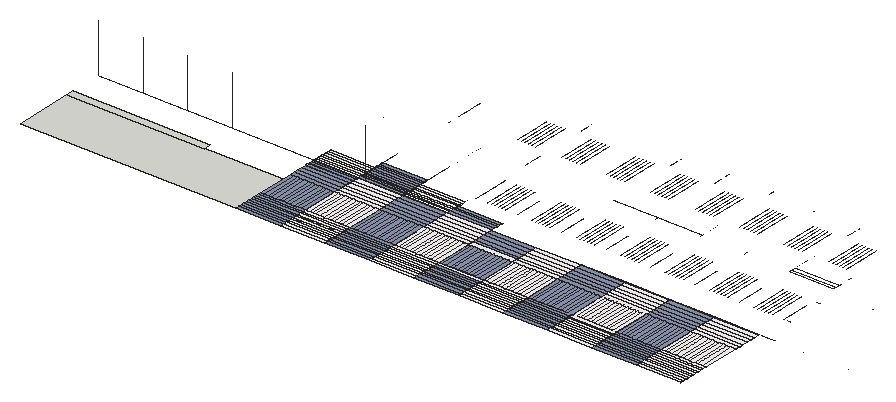
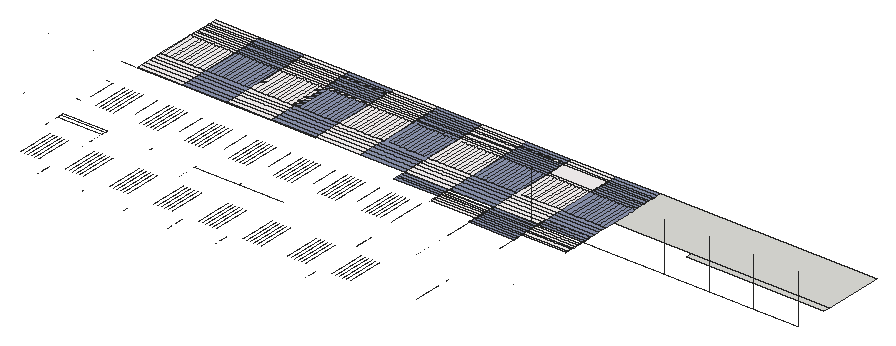
# SketchUp Ruby script. Lengths in inches.
U = 1.inch
M = Sketchup.active_model
def pt(a) = Geom::Point3d.new(a.map { |v| v * U })
def face(e, loops, mat)
  f = e.add_face(loops[0].map { |a| pt(a) })
  loops[1..].each { |l| e.add_face(l.map { |a| pt(a) }).erase! }
  f.material = f.back_material = mat if mat
  f
end
# faces: each face lists its corners as indices into pts; further lists are holes
def faces(e, pts, list, mat = nil) = list.each { |f| face(e, (f[0].is_a?(Array) ? f : [f]).map { |l| l.map { |i| pts[i] } }, mat) }
# xy, xz, yz: faces in a plane at the given z, y or x. An outline is a flat list of corners, or four numbers for a rectangle; further outlines are holes
def ring(l) = l.size == 4 ? [[l[0], l[1]], [l[2], l[1]], [l[2], l[3]], [l[0], l[3]]] : l.each_slice(2).to_a
def flat(e, list, mat, &to3) = list.each { |f| face(e, (f[0].is_a?(Array) ? f : [f]).map { |l| ring(l).map { |u, v| to3.(u, v) } }, mat) }
def xy(e, z, list, mat = nil) = flat(e, list, mat) { |x, y| [x, y, z] }
def xz(e, y, list, mat = nil) = flat(e, list, mat) { |x, z| [x, y, z] }
def yz(e, x, list, mat = nil) = flat(e, list, mat) { |y, z| [x, y, z] }
def lines(e, pts, list) = list.each { |a, b| e.add_line(pt(pts[a]), pt(pts[b])) }
# prism: a flat outline (further loops are holes) pulled along v
def prism(e, loops, v, mat = nil)
  f = face(e, loops, mat); d = Geom::Vector3d.new(v.map { |x| x * U })
  f.pushpull(f.normal.samedirection?(d) ? d.length : -d.length)
end
def box(e, o, s, mat = nil) = prism(e, [[o, [o[0] + s[0], o[1], o[2]], [o[0] + s[0], o[1] + s[1], o[2]], [o[0], o[1] + s[1], o[2]]]], [0, 0, s[2]], mat)
def at(x, y, z, deg = 0) = Geom::Transformation.translation(pt([x, y, z])) * Geom::Transformation.rotation(ORIGIN, Z_AXIS, deg.degrees)
def axes(o, x, y, z) = Geom::Transformation.new([*x, 0, *y, 0, *z, 0, *pt(o).to_a, 1])
def part(name) = M.definitions.add(name)
# library, detail: a bought-in or finely detailed component or shape, given as its bounding box
def library(name, o, s) = part(name).tap { |d| box(d.entities, o, s) }
def detail(e, o, s) = box(e.add_group.entities, o, s)
def put(e, d, t, mat = nil) = e.add_instance(d, t).tap { |i| i.material = mat if mat }
def group(e, t, mat = nil) = e.add_group.tap { |g| g.transformation = t; g.material = mat if mat }.entities
root = M.entities
M.materials.add("Niraj_Shirt").color = [144, 153, 181]
M.materials.add("[0010_Snow]").color = [255, 250, 250]
xy(root,3034.69,[[80.5,1936.0625,635.4,2086.95],[80.5,2086.95,433.875,2104.7]])
xy(root,3034.69,[[635.4,1936.0625,749.59,1945.25],[864.34,1936.0625,978.21,1945.25],[1092.96,1936.0625,1206.84,1945.25],[1321.59,1936.0625,1435.46,1945.25],[1550.21,1936.0625,1664.09,1945.25],
  [635.4,1945.25,749.59,1954.43],[864.34,1945.25,978.21,1954.43],[1092.96,1945.25,1206.84,1954.43],[1321.59,1945.25,1435.46,1954.43],[1550.21,1945.25,1664.09,1954.43],
  [635.4,1954.43,749.59,1961.9375],[864.34,1954.43,978.21,1961.9375],[[1092.84,1954.43,1092.84,1961.9375,1206.84,1961.9375,1206.84,2007.9,1092.84,2007.9,1092.84,2015.89,1092.96,2015.89,1092.96,2124.125,1206.96,2124.125,1206.96,2111.27,1207.15,2111.27,1207.15,1954.43],[1101.05,2015.89,1196.24,2111.27]],[1092.96,1954.43,1206.84,1961.9375],[1321.46,1954.43,1321.46,1961.9375,1435.46,1961.9375,1435.46,2007.9,1321.46,2007.9,1321.46,2015.89,1424.86,2015.89,1424.86,2111.27,1435.59,2111.27,1435.59,2015.89,1435.78,2015.89,1435.78,1954.43],
  [1550.21,1954.43,1664.09,1961.9375],[635.4,1961.9375,749.59,1969.45],[864.34,1961.9375,978.21,1969.45],[1092.96,1961.9375,1206.84,1969.45],[1321.59,1961.9375,1435.46,1969.45],
  [1550.21,1961.9375,1664.09,1969.45],[635.4,1969.45,749.59,1977.23],[864.34,1969.45,978.21,1977.23],[1092.96,1969.45,1206.84,1977.23],[1321.59,1969.45,1435.46,1977.23],
  [1550.21,1969.45,1664.09,1977.23],[635.4,1977.23,749.59,1985.01],[864.34,1977.23,978.21,1985.01],[1092.96,1977.23,1206.84,1985.01],[1321.59,1977.23,1435.46,1985.01],
  [1550.21,1977.23,1664.09,1985.01],[635.4,1985.01,749.59,1992.46],[864.34,1985.01,978.21,1992.46],[1092.96,1985.01,1206.84,1992.46],[1321.59,1985.01,1435.46,1992.46],
  [1550.21,1985.01,1664.09,1992.46],[635.4,1992.46,749.59,1999.91],[864.34,1992.46,978.21,1999.91],[1092.96,1992.46,1206.84,1999.91],[1321.59,1992.46,1435.46,1999.91],
  [1550.21,1992.46,1664.09,1999.91],[635.4,1999.91,749.59,2007.9],[864.34,1999.91,978.21,2007.9],[1092.96,1999.91,1206.84,2007.9],[1321.59,1999.91,1435.46,2007.9],
  [1550.21,1999.91,1664.09,2007.9],[635.4,2007.9,749.59,2015.89],[864.34,2007.9,978.21,2015.89],[1550.21,2007.9,1664.09,2015.89],[635.4,2015.89,643.8,2111.27],
  [643.8,2015.89,652.45,2111.27],[652.45,2015.89,662.47,2111.27],[662.47,2015.89,672.48,2111.27],[672.48,2015.89,682.48,2111.27],[682.48,2015.89,691.13,2111.27],
  [691.13,2015.89,700.68,2111.27],[700.68,2015.89,709.32,2111.27],[709.32,2015.89,719.31,2111.27],[719.31,2015.89,727.95,2111.27],[727.95,2015.89,738.99,2111.27],
  [738.99,2015.89,749.71,2111.27],[864.34,2015.89,872.43,2111.27],[872.43,2015.89,881.08,2111.27],[881.08,2015.89,891.1,2111.27],[891.1,2015.89,901.1,2111.27],
  [901.1,2015.89,911.11,2111.27],[911.11,2015.89,919.76,2111.27],[919.76,2015.89,929.31,2111.27],[929.31,2015.89,937.94,2111.27],[937.94,2015.89,947.93,2111.27],
  [947.93,2015.89,956.58,2111.27],[956.58,2015.89,967.61,2111.27],[967.61,2015.89,978.34,2111.27],[1092.96,2015.89,1101.05,2111.27],[1101.05,2015.89,1109.7,2111.27],
  [1109.7,2015.89,1119.72,2111.27],[1119.72,2015.89,1129.73,2111.27],[1129.73,2015.89,1139.73,2111.27],[1139.73,2015.89,1148.38,2111.27],[1148.38,2015.89,1157.93,2111.27],
  [1157.93,2015.89,1166.57,2111.27],[1166.57,2015.89,1176.56,2111.27],[1176.56,2015.89,1185.2,2111.27],[1185.2,2015.89,1196.24,2111.27],[1196.24,2015.89,1206.96,2111.27],
  [1321.59,2015.89,1329.68,2111.27],[1329.68,2015.89,1338.33,2111.27],[1338.33,2015.89,1348.35,2111.27],[1348.35,2015.89,1358.35,2111.27],[1358.35,2015.89,1368.36,2111.27],
  [1368.36,2015.89,1377.01,2111.27],[1377.01,2015.89,1386.56,2111.27],[1386.56,2015.89,1395.19,2111.27],[1395.19,2015.89,1405.18,2111.27],[1405.18,2015.89,1413.83,2111.27],
  [1413.83,2015.89,1424.86,2111.27],[1550.21,2015.89,1558.3,2111.27],[1558.3,2015.89,1566.95,2111.27],[1566.95,2015.89,1576.97,2111.27],[1576.97,2015.89,1586.98,2111.27],
  [1586.98,2015.89,1596.98,2111.27],[1596.98,2015.89,1605.63,2111.27],[1605.63,2015.89,1615.18,2111.27],[1615.18,2015.89,1623.82,2111.27],[1623.82,2015.89,1633.81,2111.27],
  [1633.81,2015.89,1642.45,2111.27],[1642.45,2015.89,1653.49,2111.27],[1653.49,2015.89,1664.21,2111.27],[635.4,2111.27,749.71,2124.125],[864.34,2111.27,978.34,2124.125],
  [1321.59,2111.27,1435.59,2124.125],[1550.21,2111.27,1664.21,2124.125],[635.4,2124.125,749.71,2134.28],[864.34,2124.125,978.34,2134.28],[1092.96,2124.125,1206.96,2134.28],
  [1321.59,2124.125,1435.59,2134.28],[1550.21,2124.125,1664.21,2134.28],[635.4,2134.28,749.71,2146.4],[864.34,2134.28,978.34,2146.4],[1092.96,2134.28,1206.96,2146.4],
  [1321.59,2134.28,1435.59,2146.4],[1550.21,2134.28,1664.21,2146.4],[635.4,2146.4,749.71,2159.46],[864.34,2146.4,978.34,2159.46],[1092.96,2146.4,1206.96,2159.46],
  [1321.59,2146.4,1435.59,2159.46],[1550.21,2146.4,1664.21,2159.46],[864.34,2159.46,978.34,2172.125],[1092.96,2159.46,1206.96,2172.125],[1321.59,2159.46,1435.59,2172.125],
  [1550.21,2159.46,1664.21,2172.125],[635.4,2160.48,749.28,2169.66],[635.4,2172.125,635.4,2178.84,749.28,2178.84,749.28,2184.66,749.59,2184.66,749.59,2178.84,749.71,2178.84,749.71,2172.125],[864.34,2172.125,978.34,2184.66],[1092.96,2172.125,1206.96,2184.66],
  [1321.59,2172.125,1435.59,2184.66],[1550.21,2172.125,1664.21,2184.66],[635.4,2178.84,749.28,2184.66],[750.03,2186.8125,863.78,2193.84],[978.84,2186.8125,1092.71,2196],
  [978.84,2196,1092.71,2205.18],[750.03,2196.31,863.78,2203.03],[750.03,2203.03,863.78,2208.84],[978.84,2205.18,1092.71,2212.6875],[750.03,2210.54,863.78,2218.05],
  [978.84,2212.6875,1092.71,2220.2],[750.03,2218.05,863.78,2225.83],[750.03,2225.83,863.78,2233.61],[750.03,2233.61,863.78,2241.06],[750.03,2241.06,863.9,2248.51],
  [750.03,2248.51,863.9,2256.5],[750.03,2256.5,863.9,2264.48]],"Niraj_Shirt")
xy(root,3034.69,[[749.59,1936.0625,749.71,1945.25],[749.71,1936.0625,750.03,1945.25],[750.03,1936.0625,863.9,1945.25],[863.9,1936.0625,864.03,1954.43],[864.03,1936.0625,864.21,1945.25],
  [864.21,1936.0625,864.34,1945.25],[978.21,1936.0625,978.34,1954.43],[978.34,1936.0625,978.53,1945.25],[978.53,1936.0625,978.65,1945.25],[978.65,1936.0625,1092.53,1945.25],
  [1092.53,1936.0625,1092.65,1954.43],[1092.65,1936.0625,1092.84,1945.25],[1092.84,1936.0625,1092.96,1945.25],[1206.84,1936.0625,1206.96,1954.43],[1206.96,1936.0625,1207.15,1945.25],
  [1207.15,1936.0625,1207.28,1945.25],[1207.28,1936.0625,1321.15,1945.25],[1321.15,1936.0625,1321.28,1954.43],[1321.28,1936.0625,1321.46,1945.25],[1321.46,1936.0625,1321.59,1945.25],
  [1435.46,1936.0625,1435.59,1954.43],[1435.59,1936.0625,1435.78,1945.25],[1435.78,1936.0625,1435.9,1945.25],[1435.9,1936.0625,1549.78,1945.25],[1549.78,1936.0625,1549.9,1954.43],
  [1549.9,1936.0625,1550.09,1945.25],[1550.09,1936.0625,1550.21,1945.25],[1664.09,1936.0625,1664.21,1954.43],[1664.21,1936.0625,1664.4,1945.25],[1664.4,1936.0625,1664.53,1945.25],
  [1664.53,1936.0625,1778.4,1945.25],[1778.4,1936.0625,1778.71,1954.43],[749.59,1945.25,749.71,1954.43],[749.71,1945.25,750.03,1954.43],[750.03,1945.25,863.9,1954.43],
  [864.03,1945.25,864.21,1954.43],[864.21,1945.25,864.34,1954.43],[978.34,1945.25,978.53,1954.43],[978.53,1945.25,978.65,1954.43],[978.65,1945.25,1092.53,1954.43],
  [1092.65,1945.25,1092.84,1954.43],[1092.84,1945.25,1092.96,1954.43],[1206.96,1945.25,1207.15,1954.43],[1207.15,1945.25,1207.28,1954.43],[1207.28,1945.25,1321.15,1954.43],
  [1321.28,1945.25,1321.46,1954.43],[1321.46,1945.25,1321.59,1954.43],[1435.59,1945.25,1435.78,1954.43],[1435.78,1945.25,1435.9,1954.43],[1435.9,1945.25,1549.78,1954.43],
  [1549.9,1945.25,1550.09,1954.43],[1550.09,1945.25,1550.21,1954.43],[1664.21,1945.25,1664.4,1954.43],[1664.4,1945.25,1664.53,1954.43],[1664.53,1945.25,1778.4,1954.43],
  [749.59,1954.43,749.71,2015.89],[749.71,1954.43,750.03,1961.9375],[750.03,1954.43,863.9,1961.9375],[863.9,1954.43,863.9,1961.9375,750.03,1961.9375,750.03,2007.9,863.9,2007.9,863.9,2015.89,853.3,2015.89,853.3,2111.27,750.03,2111.27,750.03,2124.125,864.03,2124.125,864.03,2111.27,864.21,2111.27,864.21,1954.43],[863.9,1954.43,864.03,2015.89],
  [864.03,1954.43,864.03,2015.89,864.21,2015.89,864.21,2007.9,864.34,2007.9,864.34,1954.43],[864.21,1954.43,864.21,1961.9375,978.21,1961.9375,978.21,2015.89,978.53,2015.89,978.53,1954.43],[978.21,1954.43,978.34,2015.89],[978.34,1954.43,978.65,2015.89],[978.53,1954.43,978.53,1961.9375,1092.53,1961.9375,1092.53,2007.9,978.53,2007.9,978.53,2015.89,1081.93,2015.89,1081.93,2111.27,1092.65,2111.27,1092.65,2015.89,1092.84,2015.89,1092.84,1954.43],
  [978.65,1954.43,1092.53,1961.9375],[1092.53,1954.43,1092.65,2015.89],[1092.65,1954.43,1092.96,2015.89],[1206.84,1954.43,1206.96,2015.89],[1206.96,1954.43,1206.96,2015.89,1207.15,2015.89,1207.15,2007.9,1207.28,2007.9,1207.28,1954.43],
  [1207.15,1954.43,1207.15,1961.9375,1321.15,1961.9375,1321.15,2015.89,1321.46,2015.89,1321.46,1954.43],[1207.28,1954.43,1321.15,1961.9375],[1321.15,1954.43,1321.28,2015.89],[1321.28,1954.43,1321.59,2015.89],[1321.59,1954.43,1435.46,1961.9375],
  [1435.46,1954.43,1435.59,2015.89],[1435.59,1954.43,1435.9,2015.89],[[1435.78,1954.43,1435.78,1961.9375,1549.78,1961.9375,1549.78,2007.9,1435.78,2007.9,1435.78,2015.89,1435.9,2015.89,1435.9,2124.125,1549.9,2124.125,1549.9,2111.27,1550.09,2111.27,1550.09,1954.43],[1443.99,2015.89,1539.18,2111.27]],[1435.9,1954.43,1549.78,1961.9375],[1549.78,1954.43,1549.9,2015.89],
  [1549.9,1954.43,1549.9,2015.89,1550.09,2015.89,1550.09,2007.9,1550.21,2007.9,1550.21,1961.9375,1550.09,1961.9375,1550.09,1954.43],[1550.09,1954.43,1550.21,1961.9375],[1664.09,1954.43,1664.21,2015.89],[1664.21,1954.43,1664.4,1961.9375],[1664.4,1954.43,1664.53,1961.9375],
  [1664.53,1954.43,1778.4,1961.9375],[1778.4,1954.43,1778.71,2015.89],[1778.71,1954.43,1778.84,2015.89],[749.71,1961.9375,750.03,1969.45],[750.03,1961.9375,863.9,1969.45],
  [864.21,1961.9375,864.34,1969.45],[978.53,1961.9375,978.65,1969.45],[978.65,1961.9375,1092.53,1969.45],[1092.84,1961.9375,1092.96,1969.45],[1207.15,1961.9375,1207.28,1969.45],
  [1207.28,1961.9375,1321.15,1969.45],[1321.46,1961.9375,1321.59,1969.45],[1435.78,1961.9375,1435.9,1969.45],[1435.9,1961.9375,1549.78,1969.45],[1550.09,1961.9375,1550.21,1969.45],
  [1664.21,1961.9375,1664.4,1969.45],[1664.4,1961.9375,1664.53,1969.45],[1664.53,1961.9375,1778.4,1969.45],[749.71,1969.45,750.03,1977.23],[750.03,1969.45,863.9,1977.23],
  [864.21,1969.45,864.34,1977.23],[978.53,1969.45,978.65,1977.23],[978.65,1969.45,1092.53,1977.23],[1092.84,1969.45,1092.96,1977.23],[1207.15,1969.45,1207.28,1977.23],
  [1207.28,1969.45,1321.15,1977.23],[1321.46,1969.45,1321.59,1977.23],[1435.78,1969.45,1435.9,1977.23],[1435.9,1969.45,1549.78,1977.23],[1550.09,1969.45,1550.21,1977.23],
  [1664.21,1969.45,1664.4,1977.23],[1664.4,1969.45,1664.53,1977.23],[1664.53,1969.45,1778.4,1977.23],[749.71,1977.23,750.03,1985.01],[750.03,1977.23,863.9,1985.01],
  [864.21,1977.23,864.34,1985.01],[978.53,1977.23,978.65,1985.01],[978.65,1977.23,1092.53,1985.01],[1092.84,1977.23,1092.96,1985.01],[1207.15,1977.23,1207.28,1985.01],
  [1207.28,1977.23,1321.15,1985.01],[1321.46,1977.23,1321.59,1985.01],[1435.78,1977.23,1435.9,1985.01],[1435.9,1977.23,1549.78,1985.01],[1550.09,1977.23,1550.21,1985.01],
  [1664.21,1977.23,1664.4,1985.01],[1664.4,1977.23,1664.53,1985.01],[1664.53,1977.23,1778.4,1985.01],[749.71,1985.01,750.03,1992.46],[750.03,1985.01,863.9,1992.46],
  [864.21,1985.01,864.34,1992.46],[978.53,1985.01,978.65,1992.46],[978.65,1985.01,1092.53,1992.46],[1092.84,1985.01,1092.96,1992.46],[1207.15,1985.01,1207.28,1992.46],
  [1207.28,1985.01,1321.15,1992.46],[1321.46,1985.01,1321.59,1992.46],[1435.78,1985.01,1435.9,1992.46],[1435.9,1985.01,1549.78,1992.46],[1550.09,1985.01,1550.21,1992.46],
  [1664.21,1985.01,1664.4,1992.46],[1664.4,1985.01,1664.53,1992.46],[1664.53,1985.01,1778.4,1992.46],[749.71,1992.46,750.03,1999.91],[750.03,1992.46,863.9,1999.91],
  [864.21,1992.46,864.34,1999.91],[978.53,1992.46,978.65,1999.91],[978.65,1992.46,1092.53,1999.91],[1092.84,1992.46,1092.96,1999.91],[1207.15,1992.46,1207.28,1999.91],
  [1207.28,1992.46,1321.15,1999.91],[1321.46,1992.46,1321.59,1999.91],[1435.78,1992.46,1435.9,1999.91],[1435.9,1992.46,1549.78,1999.91],[1550.09,1992.46,1550.21,1999.91],
  [1664.21,1992.46,1664.4,1999.91],[1664.4,1992.46,1664.53,1999.91],[1664.53,1992.46,1778.4,1999.91],[749.71,1999.91,750.03,2007.9],[750.03,1999.91,863.9,2007.9],
  [864.21,1999.91,864.34,2007.9],[978.53,1999.91,978.65,2007.9],[978.65,1999.91,1092.53,2007.9],[1092.84,1999.91,1092.96,2007.9],[1207.15,1999.91,1207.28,2007.9],
  [1207.28,1999.91,1321.15,2007.9],[1321.46,1999.91,1321.59,2007.9],[1435.78,1999.91,1435.9,2007.9],[1435.9,1999.91,1549.78,2007.9],[1550.09,1999.91,1550.21,2007.9],
  [1664.21,1999.91,1664.4,2007.9],[1664.4,1999.91,1664.53,2007.9],[1664.53,1999.91,1778.4,2007.9],[749.71,2007.9,750.03,2015.89],[750.03,2007.9,863.9,2015.89],
  [864.21,2007.9,864.34,2015.89],[978.65,2007.9,1092.53,2015.89],[1092.96,2007.9,1206.84,2015.89],[1207.15,2007.9,1207.28,2015.89],[1207.28,2007.9,1321.15,2015.89],
  [1321.59,2007.9,1435.46,2015.89],[1435.9,2007.9,1549.78,2015.89],[1550.09,2007.9,1550.21,2015.89],[1664.21,2007.9,1664.4,2015.89],[1664.4,2007.9,1664.53,2015.89],
  [1664.53,2007.9,1778.4,2015.89],[749.71,2015.89,750.03,2111.27],[750.03,2015.89,758.12,2111.27],[758.12,2015.89,766.76,2111.27],[766.76,2015.89,776.78,2111.27],
  [776.78,2015.89,786.79,2111.27],[786.79,2015.89,796.79,2111.27],[796.79,2015.89,805.45,2111.27],[805.45,2015.89,815,2111.27],[815,2015.89,823.63,2111.27],
  [823.63,2015.89,833.62,2111.27],[833.62,2015.89,842.27,2111.27],[842.27,2015.89,853.3,2111.27],[853.3,2015.89,864.03,2111.27],[864.03,2015.89,864.21,2111.27],
  [864.21,2015.89,864.34,2111.27],[978.34,2015.89,978.53,2111.27],[978.53,2015.89,978.65,2111.27],[978.65,2015.89,986.74,2111.27],[986.74,2015.89,995.39,2111.27],
  [995.39,2015.89,1005.41,2111.27],[1005.41,2015.89,1015.42,2111.27],[1015.42,2015.89,1025.42,2111.27],[1025.42,2015.89,1034.07,2111.27],[1034.07,2015.89,1043.62,2111.27],
  [1043.62,2015.89,1052.25,2111.27],[1052.25,2015.89,1062.25,2111.27],[1062.25,2015.89,1070.89,2111.27],[1070.89,2015.89,1081.93,2111.27],[1081.93,2015.89,1092.65,2111.27],
  [1092.65,2015.89,1092.84,2111.27],[1092.84,2015.89,1092.96,2111.27],[1206.96,2015.89,1207.15,2111.27],[1207.15,2015.89,1207.28,2111.27],[1207.28,2015.89,1215.37,2111.27],
  [1215.37,2015.89,1224.01,2111.27],[1224.01,2015.89,1234.03,2111.27],[1234.03,2015.89,1244.04,2111.27],[1244.04,2015.89,1254.04,2111.27],[1254.04,2015.89,1262.7,2111.27],
  [1262.7,2015.89,1272.25,2111.27],[1272.25,2015.89,1280.88,2111.27],[1280.88,2015.89,1290.87,2111.27],[1290.87,2015.89,1299.52,2111.27],[1299.52,2015.89,1310.55,2111.27],
  [1310.55,2015.89,1321.28,2111.27],[1321.28,2015.89,1321.46,2111.27],[1321.46,2015.89,1321.59,2111.27],[1424.86,2015.89,1435.59,2111.27],[1435.59,2015.89,1435.78,2111.27],
  [1435.78,2015.89,1435.9,2111.27],[1435.9,2015.89,1443.99,2111.27],[1443.99,2015.89,1452.64,2111.27],[1452.64,2015.89,1462.66,2111.27],[1462.66,2015.89,1472.67,2111.27],
  [1472.67,2015.89,1482.67,2111.27],[1482.67,2015.89,1491.32,2111.27],[1491.32,2015.89,1500.87,2111.27],[1500.87,2015.89,1509.5,2111.27],[1509.5,2015.89,1519.5,2111.27],
  [1519.5,2015.89,1528.14,2111.27],[1528.14,2015.89,1539.18,2111.27],[1539.18,2015.89,1549.9,2111.27],[1549.9,2015.89,1550.09,2111.27],[1550.09,2015.89,1550.21,2111.27],
  [1664.21,2015.89,1664.4,2111.27],[1664.4,2015.89,1664.53,2111.27],[1664.53,2015.89,1672.62,2111.27],[1672.62,2015.89,1681.26,2111.27],[1681.26,2015.89,1691.28,2111.27],
  [1691.28,2015.89,1701.29,2111.27],[1701.29,2015.89,1711.29,2111.27],[1711.29,2015.89,1719.95,2111.27],[1719.95,2015.89,1729.5,2111.27],[1729.5,2015.89,1738.13,2111.27],
  [1738.13,2015.89,1748.12,2111.27],[1748.12,2015.89,1756.77,2111.27],[1756.77,2015.89,1767.8,2111.27],[1767.8,2015.89,1778.71,2111.27],[1778.71,2015.89,1778.84,2111.27],
  [749.71,2111.27,750.03,2124.125],[750.03,2111.27,864.03,2124.125],[864.03,2111.27,864.21,2124.125],[864.21,2111.27,864.34,2124.125],[978.34,2111.27,978.53,2124.125],
  [978.53,2111.27,978.65,2124.125],[978.65,2111.27,1092.65,2124.125],[1092.65,2111.27,1092.84,2124.125],[1092.84,2111.27,1092.96,2124.125],[1092.96,2111.27,1206.96,2124.125],
  [1206.96,2111.27,1207.15,2124.125],[1207.15,2111.27,1207.28,2124.125],[1207.28,2111.27,1321.28,2124.125],[1321.28,2111.27,1321.46,2124.125],[1321.46,2111.27,1321.59,2124.125],
  [1435.59,2111.27,1435.78,2124.125],[1435.78,2111.27,1435.9,2124.125],[1435.9,2111.27,1549.9,2124.125],[1549.9,2111.27,1550.09,2124.125],[1550.09,2111.27,1550.21,2124.125],
  [1664.21,2111.27,1664.4,2124.125],[1664.4,2111.27,1664.53,2124.125],[1664.53,2111.27,1778.71,2124.125],[1778.71,2111.27,1778.84,2124.125],[749.71,2124.125,750.03,2134.28],
  [750.03,2124.125,864.03,2134.28],[864.03,2124.125,864.21,2134.28],[864.21,2124.125,864.34,2134.28],[978.34,2124.125,978.53,2134.28],[978.53,2124.125,978.65,2134.28],
  [978.65,2124.125,1092.65,2134.28],[1092.65,2124.125,1092.84,2134.28],[1092.84,2124.125,1092.96,2134.28],[1206.96,2124.125,1207.15,2134.28],[1207.15,2124.125,1207.28,2134.28],
  [1207.28,2124.125,1321.28,2134.28],[1321.28,2124.125,1321.46,2134.28],[1321.46,2124.125,1321.59,2134.28],[1435.59,2124.125,1435.78,2134.28],[1435.78,2124.125,1435.9,2134.28],
  [1435.9,2124.125,1549.9,2134.28],[1549.9,2124.125,1550.09,2134.28],[1550.09,2124.125,1550.21,2134.28],[1664.21,2124.125,1664.4,2134.28],[1664.4,2124.125,1664.53,2134.28],
  [1664.53,2124.125,1778.71,2134.28],[1778.71,2124.125,1778.84,2134.28],[749.71,2134.28,750.03,2146.4],[750.03,2134.28,864.03,2146.4],[864.03,2134.28,864.21,2146.4],
  [864.21,2134.28,864.34,2146.4],[978.34,2134.28,978.53,2146.4],[978.53,2134.28,978.65,2146.4],[978.65,2134.28,1092.65,2146.4],[1092.65,2134.28,1092.84,2146.4],
  [1092.84,2134.28,1092.96,2146.4],[1206.96,2134.28,1207.15,2146.4],[1207.15,2134.28,1207.28,2146.4],[1207.28,2134.28,1321.28,2146.4],[1321.28,2134.28,1321.46,2146.4],
  [1321.46,2134.28,1321.59,2146.4],[1435.59,2134.28,1435.78,2146.4],[1435.78,2134.28,1435.9,2146.4],[1435.9,2134.28,1549.9,2146.4],[1549.9,2134.28,1550.09,2146.4],
  [1550.09,2134.28,1550.21,2146.4],[1664.21,2134.28,1664.4,2146.4],[1664.4,2134.28,1664.53,2146.4],[1664.53,2134.28,1778.71,2146.4],[1778.71,2134.28,1778.84,2146.4],
  [749.71,2146.4,750.03,2159.46],[750.03,2146.4,864.03,2159.46],[864.03,2146.4,864.21,2159.46],[864.21,2146.4,864.34,2159.46],[978.34,2146.4,978.53,2159.46],
  [978.53,2146.4,978.65,2159.46],[978.65,2146.4,1092.65,2159.46],[1092.65,2146.4,1092.84,2159.46],[1092.84,2146.4,1092.96,2159.46],[1206.96,2146.4,1207.15,2159.46],
  [1207.15,2146.4,1207.28,2159.46],[1207.28,2146.4,1321.28,2159.46],[1321.28,2146.4,1321.46,2159.46],[1321.46,2146.4,1321.59,2159.46],[1435.59,2146.4,1435.78,2159.46],
  [1435.78,2146.4,1435.9,2159.46],[1435.9,2146.4,1549.9,2159.46],[1549.9,2146.4,1550.09,2159.46],[1550.09,2146.4,1550.21,2159.46],[1664.21,2146.4,1664.4,2159.46],
  [1664.4,2146.4,1664.53,2159.46],[1664.53,2146.4,1778.71,2159.46],[1778.71,2146.4,1778.84,2159.46],[635.4,2159.46,749.71,2160.48],[749.71,2159.46,750.03,2172.125],
  [750.03,2159.46,864.03,2172.125],[864.03,2159.46,864.21,2172.125],[864.21,2159.46,864.34,2172.125],[978.34,2159.46,978.53,2172.125],[978.53,2159.46,978.65,2172.125],
  [978.65,2159.46,1092.65,2172.125],[1092.65,2159.46,1092.84,2172.125],[1092.84,2159.46,1092.96,2172.125],[1206.96,2159.46,1207.15,2172.125],[1207.15,2159.46,1207.28,2172.125],
  [1207.28,2159.46,1321.28,2172.125],[1321.28,2159.46,1321.46,2172.125],[1321.46,2159.46,1321.59,2172.125],[1435.59,2159.46,1435.78,2172.125],[1435.78,2159.46,1435.9,2172.125],
  [1435.9,2159.46,1549.9,2172.125],[1549.9,2159.46,1550.09,2172.125],[1550.09,2159.46,1550.21,2172.125],[1664.21,2159.46,1664.4,2172.125],[1664.4,2159.46,1664.53,2172.125],
  [1664.53,2159.46,1778.71,2172.125],[1778.71,2159.46,1778.84,2172.125],[634.96,2160.48,635.09,2169.66],[635.09,2160.48,635.4,2169.66],[749.28,2160.48,749.28,2172.125,749.59,2172.125,749.59,2169.66,749.4,2169.66,749.4,2160.48],
  [749.28,2160.48,749.4,2178.84],[749.4,2160.48,749.59,2169.66],[749.59,2160.48,749.71,2169.66],[634.96,2169.66,635.09,2178.84],[635.09,2169.66,635.4,2178.84],
  [635.4,2169.66,749.28,2172.125],[749.4,2169.66,749.59,2178.84],[749.59,2169.66,749.71,2172.125],[635.4,2172.125,749.28,2178.84],[749.59,2172.125,749.71,2178.84],
  [749.71,2172.125,750.03,2184.66],[750.03,2172.125,864.03,2184.66],[864.03,2172.125,864.21,2184.66],[864.21,2172.125,864.34,2184.66],[978.34,2172.125,978.53,2184.66],
  [978.53,2172.125,978.65,2184.66],[978.65,2172.125,1092.65,2184.66],[1092.65,2172.125,1092.84,2184.66],[1092.84,2172.125,1092.96,2184.66],[1206.96,2172.125,1207.15,2184.66],
  [1207.15,2172.125,1207.28,2184.66],[1207.28,2172.125,1321.28,2184.66],[1321.28,2172.125,1321.46,2184.66],[1321.46,2172.125,1321.59,2184.66],[1435.59,2172.125,1435.78,2184.66],
  [1435.78,2172.125,1435.9,2184.66],[1435.9,2172.125,1549.9,2184.66],[1549.9,2172.125,1550.09,2184.66],[1550.09,2172.125,1550.21,2184.66],[1664.21,2172.125,1664.4,2184.66],
  [1664.4,2172.125,1664.53,2184.66],[1664.53,2172.125,1778.71,2184.66],[1778.71,2172.125,1778.84,2184.66],[634.96,2178.84,635.09,2186.8125],[635.09,2178.84,635.4,2186.35],
  [749.28,2178.84,749.4,2186.8125],[749.4,2178.84,749.59,2186.35],[749.59,2178.84,749.71,2184.66],[635.4,2184.66,749.28,2186.35],[749.28,2184.66,749.28,2186.8125,749.4,2186.8125,749.4,2186.35,749.59,2186.35,749.59,2184.66],
  [749.59,2184.66,749.71,2186.35],[749.71,2184.66,750.03,2186.8125],[863.9,2184.66,864.03,2185.53],[864.03,2184.66,864.21,2185.53],[864.21,2184.66,864.34,2185.53],
  [864.34,2184.66,978.53,2185.53],[1321.46,2184.66,1435.78,2186.8125],[1435.78,2184.66,1550.09,2186.8125],[1550.09,2184.66,1664.4,2186.8125],[1664.4,2184.66,1778.71,2186.8125],
  [863.9,2185.53,864.03,2186.8125],[864.03,2185.53,864.21,2186.8125],[864.21,2185.53,864.34,2186.8125],[864.34,2185.53,977.9,2186.8125],[977.9,2185.53,978.09,2186.8125],
  [978.09,2185.53,978.21,2186.8125],[978.21,2185.53,978.4,2186.8125],[978.4,2185.53,978.53,2186.8125],[635.09,2186.35,635.4,2186.8125],[635.4,2186.35,749.28,2186.8125],
  [749.4,2186.35,749.59,2186.8125],[749.59,2186.35,749.71,2186.8125],[863.78,2187.23,863.9,2192.07],[863.78,2192.07,863.9,2193.84],[864.03,2192.07,864.21,2193.84],
  [864.21,2192.07,864.34,2193.84],[978.09,2192.07,978.21,2203.9],[749.59,2193.84,749.71,2193.87],[749.71,2193.84,750.03,2203.03],[750.03,2193.84,863.78,2196.31],
  [863.78,2193.84,863.9,2194.72],[864.03,2193.84,864.21,2194.72],[864.21,2193.84,864.34,2194.72],[635.09,2193.87,635.4,2201.65],[635.4,2193.87,749.28,2201.65],
  [749.4,2193.87,749.59,2201.65],[749.59,2193.87,749.71,2201.65],[863.78,2194.72,863.9,2194.74],[863.9,2194.72,864.03,2203.03],[864.03,2194.72,864.21,2203.03],
  [864.21,2194.72,864.34,2196.31],[864.34,2194.72,978.09,2197.18],[978.21,2194.72,978.4,2203.9],[978.4,2194.72,978.53,2197.18],[863.78,2194.74,863.9,2196.31],
  [863.78,2196.31,863.9,2202.52],[864.21,2196.31,864.34,2197.18],[864.21,2197.18,864.34,2203.03],[864.34,2197.18,978.09,2203.9],[978.4,2197.18,978.53,2203.9],
  [635.09,2201.65,635.4,2209.43],[635.4,2201.65,749.28,2209.43],[749.4,2201.65,749.59,2209.43],[749.59,2201.65,749.71,2203.03],[863.78,2202.52,863.9,2203.03],
  [749.59,2203.03,749.71,2209.43],[749.71,2203.03,750.03,2210.54],[863.78,2203.03,863.9,2208.84],[863.9,2203.03,864.03,2203.9],[864.03,2203.03,864.21,2203.9],
  [864.21,2203.03,864.34,2203.9],[863.9,2203.9,864.03,2211.41],[864.03,2203.9,864.21,2210.54],[864.21,2203.9,864.34,2209.72],[864.34,2203.9,978.09,2209.72],
  [978.4,2203.9,978.53,2211.41],[750.03,2208.84,863.78,2210.54],[863.78,2208.84,863.9,2210.54],[635.09,2209.43,635.4,2216.875],[635.4,2209.43,749.28,2216.875],
  [749.4,2209.43,749.59,2216.875],[749.59,2209.43,749.71,2216.875],[864.21,2209.72,864.34,2210.54],[864.34,2209.72,978.09,2211.41],[749.71,2210.54,750.03,2218.05],
  [863.78,2210.54,863.9,2217.75],[864.03,2210.54,864.21,2211.41],[864.21,2210.54,864.34,2211.41],[863.9,2211.41,864.03,2218.92],[864.03,2211.41,864.21,2218.05],
  [864.21,2211.41,864.34,2218.05],[864.34,2211.41,978.09,2218.92],[978.4,2211.41,978.53,2218.92],[635.09,2216.875,635.4,2224.32],[635.4,2216.875,749.28,2224.32],
  [749.4,2216.875,749.59,2224.32],[749.59,2216.875,749.71,2224.32],[863.78,2217.75,863.9,2218.05],[749.71,2218.05,750.03,2225.83],[863.78,2218.05,863.9,2218.92],
  [864.03,2218.05,864.21,2218.92],[864.21,2218.05,864.34,2218.92],[863.78,2218.92,863.9,2225.2],[863.9,2218.92,864.03,2226.7],[864.03,2218.92,864.21,2225.83],
  [864.21,2218.92,864.34,2225.83],[864.34,2218.92,978.09,2226.7],[978.4,2218.92,978.53,2226.7],[635.09,2224.32,635.4,2232.3125],[635.4,2224.32,749.28,2232.3125],
  [749.4,2224.32,749.59,2232.3125],[749.59,2224.32,749.71,2232.3125],[863.78,2225.2,863.9,2225.83],[749.71,2225.83,750.03,2233.61],[863.78,2225.83,863.9,2233.61],
  [864.03,2225.83,864.21,2226.7],[864.21,2225.83,864.34,2226.7],[863.9,2226.7,864.03,2234.48],[864.03,2226.7,864.21,2233.61],[864.21,2226.7,864.34,2233.61],
  [864.34,2226.7,978.09,2234.48],[978.4,2226.7,978.53,2234.48],[635.09,2232.3125,635.4,2240.3],[635.4,2232.3125,749.28,2240.3],[749.4,2232.3125,749.59,2240.3],
  [749.59,2232.3125,749.71,2240.3],[749.71,2233.61,750.03,2241.06],[863.78,2233.61,863.9,2241.06],[864.03,2233.61,864.21,2234.48],[864.21,2233.61,864.34,2234.48],
  [863.9,2234.48,864.03,2241.93],[864.03,2234.48,864.21,2241.06],[864.21,2234.48,864.34,2241.06],[864.34,2234.48,978.09,2241.93],[978.4,2234.48,978.53,2241.93],
  [749.59,2240.3,749.71,2264.48],[749.71,2241.06,750.03,2248.51],[864.03,2241.06,864.21,2241.93],[864.21,2241.06,864.34,2241.93],[863.9,2241.93,864.03,2249.38],
  [864.03,2241.93,864.21,2248.51],[864.21,2241.93,864.34,2248.51],[749.71,2248.51,750.03,2256.5],[864.03,2248.51,864.21,2249.38],[864.21,2248.51,864.34,2249.38],
  [863.9,2249.38,864.03,2257.37],[864.03,2249.38,864.21,2256.5],[864.21,2249.38,864.34,2256.5],[749.71,2256.5,750.03,2264.48],[864.03,2256.5,864.21,2257.37],
  [864.21,2256.5,864.34,2257.37],[863.9,2257.37,864.03,2264.48],[864.03,2257.37,864.21,2264.48],[864.21,2257.37,864.34,2264.48],[863.9,2264.48,864.03,2265.36],
  [864.03,2264.48,864.21,2265.36],[864.21,2264.48,864.34,2265.36]],"[0010_Snow]")
p = [[863.9,2015.89,3034.69],[863.9,2086.95,3034.69],[864.03,1999.91,3034.69],[864.21,1999.91,3034.69],[864.03,1969.45,3034.69],[864.21,1969.45,3034.69],
  [864.03,1985.01,3034.69],[864.21,1985.01,3034.69],[864.21,1961.9375,3034.69],[864.03,1961.9375,3034.69],[864.21,1977.23,3034.69],[864.03,1977.23,3034.69],
  [864.21,1992.46,3034.69],[864.03,1992.46,3034.69],[864.21,2007.9,3034.69],[864.03,2007.9,3034.69],[978.21,2015.89,3034.69],[978.21,2086.95,3034.69],
  [978.34,1999.91,3034.69],[978.53,1999.91,3034.69],[978.34,1969.45,3034.69],[978.53,1969.45,3034.69],[978.34,1985.01,3034.69],[978.53,1985.01,3034.69],
  [978.53,1961.9375,3034.69],[978.34,1961.9375,3034.69],[978.53,1977.23,3034.69],[978.34,1977.23,3034.69],[978.53,1992.46,3034.69],[978.34,1992.46,3034.69],
  [978.53,2007.9,3034.69],[978.34,2007.9,3034.69],[1092.53,2015.89,3034.69],[1092.53,2086.95,3034.69],[1092.65,1999.91,3034.69],[1092.84,1999.91,3034.69],
  [1092.65,1969.45,3034.69],[1092.84,1969.45,3034.69],[1092.65,1985.01,3034.69],[1092.84,1985.01,3034.69],[1092.84,1961.9375,3034.69],[1092.65,1961.9375,3034.69],
  [1092.84,1977.23,3034.69],[1092.65,1977.23,3034.69],[1092.84,1992.46,3034.69],[1092.65,1992.46,3034.69],[1092.84,2007.9,3034.69],[1092.65,2007.9,3034.69],
  [1206.84,2015.89,3034.69],[1206.84,2086.95,3034.69],[1206.96,1999.91,3034.69],[1207.15,1999.91,3034.69],[1206.96,1969.45,3034.69],[1207.15,1969.45,3034.69],
  [1206.96,1985.01,3034.69],[1207.15,1985.01,3034.69],[1207.15,1961.9375,3034.69],[1206.96,1961.9375,3034.69],[1207.15,1977.23,3034.69],[1206.96,1977.23,3034.69],
  [1207.15,1992.46,3034.69],[1206.96,1992.46,3034.69],[1207.15,2007.9,3034.69],[1206.96,2007.9,3034.69],[1321.15,2015.89,3034.69],[1321.15,2086.95,3034.69],
  [1321.28,1999.91,3034.69],[1321.46,1999.91,3034.69],[1321.28,1969.45,3034.69],[1321.46,1969.45,3034.69],[1321.28,1985.01,3034.69],[1321.46,1985.01,3034.69],
  [1321.46,1961.9375,3034.69],[1321.28,1961.9375,3034.69],[1321.46,1977.23,3034.69],[1321.28,1977.23,3034.69],[1321.46,1992.46,3034.69],[1321.28,1992.46,3034.69],
  [1321.46,2007.9,3034.69],[1321.28,2007.9,3034.69],[1435.46,2015.89,3034.69],[1435.46,2086.95,3034.69],[1435.59,1999.91,3034.69],[1435.78,1999.91,3034.69],
  [1435.59,1969.45,3034.69],[1435.78,1969.45,3034.69],[1435.59,1985.01,3034.69],[1435.78,1985.01,3034.69],[1435.78,1961.9375,3034.69],[1435.59,1961.9375,3034.69],
  [1435.78,1977.23,3034.69],[1435.59,1977.23,3034.69],[1435.78,1992.46,3034.69],[1435.59,1992.46,3034.69],[1435.78,2007.9,3034.69],[1435.59,2007.9,3034.69],
  [1549.78,2015.89,3034.69],[1549.78,2086.95,3034.69],[1549.9,1999.91,3034.69],[1550.09,1999.91,3034.69],[1549.9,1969.45,3034.69],[1550.09,1969.45,3034.69],
  [1549.9,1985.01,3034.69],[1550.09,1985.01,3034.69],[1550.09,1961.9375,3034.69],[1549.9,1961.9375,3034.69],[1550.09,1977.23,3034.69],[1549.9,1977.23,3034.69],
  [1550.09,1992.46,3034.69],[1549.9,1992.46,3034.69],[1550.09,2007.9,3034.69],[1549.9,2007.9,3034.69],[1664.09,2015.89,3034.69],[1664.09,2086.95,3034.69],
  [978.4,2211.41,3034.69],[978.21,2211.41,3034.69],[863.78,2185.53,3034.69],[863.78,2186.8125,3034.69],[978.4,2226.7,3034.69],[978.21,2226.7,3034.69],
  [863.78,2241.06,3034.69],[863.78,2241.17,3034.69],[978.4,2241.93,3034.69],[978.21,2241.93,3034.69],[978.21,2218.92,3034.69],[978.4,2218.92,3034.69],
  [978.21,2234.48,3034.69],[978.4,2234.48,3034.69],[80.6875,2186.8125,3034.69],[195,2186.8125,3034.69],[80.6875,2186.8125,3161.9375],[309.3125,2186.8125,3034.69],
  [195,2186.8125,3161.9375],[423.625,2186.8125,3034.69],[309.3125,2186.8125,3161.9375],[1321.34,2266.64,3034.69],[1321.34,2337.7,3034.69],[1291.06,2362.02,3034.69],
  [1291.06,2266.64,3034.69],[433.875,2186.8125,3034.69],[423.625,2186.8125,3161.9375],[1435.65,2266.64,3034.69],[1435.65,2337.7,3034.69],[1395.38,2362.02,3034.69],
  [1395.38,2266.64,3034.69],[1358.54,2362.02,3034.69],[1358.54,2266.64,3034.69],[1368.54,2362.02,3034.69],[1368.54,2266.64,3034.69],[1377.2,2362.02,3034.69],
  [1377.2,2266.64,3034.69],[1405.37,2362.02,3034.69],[1405.37,2266.64,3034.69],[1386.75,2362.02,3034.69],[1386.75,2266.64,3034.69],[548.1875,2186.8125,3034.69],
  [1549.96,2266.64,3034.69],[1549.96,2337.7,3034.69],[634.96,2186.8125,3034.69],[1664.28,2266.64,3034.69],[1664.28,2337.7,3034.69],[1624,2362.02,3034.69],
  [1624,2266.64,3034.69],[1587.17,2362.02,3034.69],[1587.17,2266.64,3034.69],[1597.17,2362.02,3034.69],[1597.17,2266.64,3034.69],[1605.82,2362.02,3034.69],
  [1605.82,2266.64,3034.69],[1634,2362.02,3034.69],[1634,2266.64,3034.69],[1615.37,2362.02,3034.69],[1615.37,2266.64,3034.69],[766.5625,2186.8125,3034.69],
  [766.5625,2186.8125,3161.9375],[1778.59,2266.64,3034.69],[1778.59,2337.7,3034.69],[1738.32,2362.02,3034.69],[1738.32,2266.64,3034.69],[1701.48,2362.02,3034.69],
  [1701.48,2266.64,3034.69],[1711.48,2362.02,3034.69],[1711.48,2266.64,3034.69],[1720.13,2362.02,3034.69],[1720.13,2266.64,3034.69],[1748.31,2362.02,3034.69],
  [1748.31,2266.64,3034.69],[1729.68,2362.02,3034.69],[1729.68,2266.64,3034.69],[1893.03,2409.08,3034.69],[1893.03,2410.21,3034.69],[1892.9,2186.8125,3034.69],
  [1893.03,2186.8125,3034.69],[1893.21,2186.8125,3034.69],[1893.34,2186.8125,3034.69],[2007.21,2186.8125,3034.69],[2007.34,2186.8125,3034.69],[2007.53,2186.8125,3034.69],
  [2007.65,2186.8125,3034.69],[1795.76,2362.02,3034.69],[1787.12,2362.02,3034.69],[1787.12,2266.64,3034.69],[1795.76,2266.64,3034.69],[1892.71,2409.08,3034.69],
  [1784.73,2186.8125,3034.69],[1819.79,2186.8125,3034.69],[1501.06,2362.02,3034.69],[1501.06,2266.64,3034.69],[1509.69,2362.02,3034.69],[1509.69,2266.64,3034.69],
  [1482.86,2362.02,3034.69],[1482.86,2266.64,3034.69],[1491.51,2362.02,3034.69],[1491.51,2266.64,3034.69],[1519.68,2362.02,3034.69],[1519.68,2266.64,3034.69],
  [1472.85,2362.02,3034.69],[1472.85,2266.64,3034.69],[1092.71,2266.64,3034.69],[1092.71,2337.7,3034.69],[1052.44,2362.02,3034.69],[1052.44,2266.64,3034.69],
  [986.93,2362.02,3034.69],[986.93,2266.64,3034.69],[1015.6,2362.02,3034.69],[1015.6,2266.64,3034.69],[1025.61,2362.02,3034.69],[1025.61,2266.64,3034.69],
  [1034.26,2362.02,3034.69],[1034.26,2266.64,3034.69],[1062.43,2362.02,3034.69],[1062.43,2266.64,3034.69],[1043.81,2362.02,3034.69],[1043.81,2266.64,3034.69],
  [634.96,2409.08,3034.69],[635.09,2409.08,3034.69],[749.28,2240.3,3034.69],[749.28,2311.37,3034.69],[749.9,2475.68,3034.69],[749.9,2482.37,3034.69],
  [749.71,2506.55,3034.69],[749.71,2577.62,3034.69],[863.9,2265.36,3034.69],[863.9,2335.55,3034.69],[864.03,2408.94,3034.69],[863.9,2408.94,3034.69],
  [864.03,2395.87,3034.69],[863.9,2395.87,3034.69],[863.9,2427.6,3034.69],[864.03,2427.6,3034.69],[863.9,2434.13,3034.69],[864.03,2434.13,3034.69],
  [863.9,2421.59,3034.69],[864.03,2421.59,3034.69],[978.21,2249.38,3034.69],[978.4,2249.38,3034.69],[863.9,2409.95,3034.69],[864.03,2409.95,3034.69],
  [864.03,2360.74,3034.69],[863.9,2360.74,3034.69],[1262.88,2362.02,3034.69],[1262.88,2266.64,3034.69],[1281.07,2362.02,3034.69],[1281.07,2266.64,3034.69],
  [1272.43,2362.02,3034.69],[1272.43,2266.64,3034.69],[1254.23,2362.02,3034.69],[1254.23,2266.64,3034.69],[1244.23,2362.02,3034.69],[1244.23,2266.64,3034.69],
  [1176.75,2362.02,3034.69],[1176.75,2266.64,3034.69],[1139.92,2362.02,3034.69],[1139.92,2266.64,3034.69],[1166.75,2362.02,3034.69],[1166.75,2266.64,3034.69],
  [1148.57,2362.02,3034.69],[1148.57,2266.64,3034.69],[1158.12,2362.02,3034.69],[1158.12,2266.64,3034.69],[1207.03,2266.64,3034.69],[1207.03,2337.7,3034.69],
  [1129.92,2362.02,3034.69],[1129.92,2266.64,3034.69],[947.93,2601.94,3034.69],[947.93,2506.55,3034.69],[911.11,2601.94,3034.69],[911.11,2506.55,3034.69],
  [937.94,2601.94,3034.69],[937.94,2506.55,3034.69],[919.76,2601.94,3034.69],[919.76,2506.55,3034.69],[929.31,2601.94,3034.69],[929.31,2506.55,3034.69],
  [901.1,2601.94,3034.69],[901.1,2506.55,3034.69],[978.96,2624.95,3034.69],[978.96,2614.79,3034.69],[1062.56,2601.94,3034.69],[1062.56,2506.55,3034.69],
  [978.96,2460.12,3034.69],[978.96,2452.6,3034.69],[979.15,2460.12,3034.69],[978.96,2475.68,3034.69],[978.96,2467.9,3034.69],[979.15,2475.68,3034.69],
  [978.96,2637.0625,3034.69],[978.96,2483.125,3034.69],[1043.93,2601.94,3034.69],[1043.93,2506.55,3034.69],[1052.57,2601.94,3034.69],[1052.57,2506.55,3034.69],
  [978.96,2445.09,3034.69],[978.96,2438.375,3034.69],[1015.73,2601.94,3034.69],[1015.73,2506.55,3034.69],[1025.73,2601.94,3034.69],[1025.73,2506.55,3034.69],
  [978.96,2649,3034.69],[979.15,2649,3034.69],[1034.38,2601.94,3034.69],[1034.38,2506.55,3034.69],[979.15,2445.09,3034.69],[979.28,2445.09,3034.69],
  [979.28,2637.0625,3034.69],[979.15,2637.0625,3034.69],[979.28,2460.12,3034.69],[979.28,2475.68,3034.69],[979.15,2624.95,3034.69],[978.96,2435.91,3034.69],
  [979.28,2649,3034.69],[979.28,2624.95,3034.69],[979.28,2452.6,3034.69],[979.15,2452.6,3034.69],[979.28,2467.9,3034.69],[979.15,2467.9,3034.69],
  [1176.56,2601.94,3034.69],[1176.56,2506.55,3034.69],[1139.73,2601.94,3034.69],[1139.73,2506.55,3034.69],[1148.38,2601.94,3034.69],[1148.38,2506.55,3034.69],
  [1166.57,2601.94,3034.69],[1166.57,2506.55,3034.69],[1129.73,2601.94,3034.69],[1129.73,2506.55,3034.69],[1157.93,2601.94,3034.69],[1157.93,2506.55,3034.69],
  [1207.46,2650.13,3034.69],[1207.28,2650.13,3034.69],[1207.59,2637.0625,3034.69],[1207.46,2637.0625,3034.69],[1207.46,2624.95,3034.69],[1207.28,2624.95,3034.69],
  [1321.03,2426.73,3034.69],[1321.03,2434.13,3034.69],[1207.28,2637.0625,3034.69],[1207.46,2651.15,3034.69],[1207.59,2651.15,3034.69],[1207.59,2650.13,3034.69],
  [1207.59,2434.13,3034.69],[1290.87,2601.94,3034.69],[1290.87,2506.55,3034.69],[1207.28,2614.79,3034.69],[1207.28,2649,3034.69],[1207.46,2649,3034.69],
  [1244.04,2601.94,3034.69],[1244.04,2506.55,3034.69],[1207.59,2624.95,3034.69],[1207.59,2649,3034.69],[1254.04,2601.94,3034.69],[1254.04,2506.55,3034.69],
  [1262.7,2601.94,3034.69],[1262.7,2506.55,3034.69],[1280.88,2601.94,3034.69],[1280.88,2506.55,3034.69],[1272.25,2601.94,3034.69],[1272.25,2506.55,3034.69],
  [1321.28,2650.13,3034.69],[1321.28,2662.79,3034.69],[1321.9,2637.0625,3034.69],[1321.78,2637.0625,3034.69],[1321.78,2650.13,3034.69],[1321.59,2650.13,3034.69],
  [1435.34,2426.73,3034.69],[1435.34,2434.13,3034.69],[1321.78,2624.95,3034.69],[1321.59,2624.95,3034.69],[1321.59,2637.0625,3034.69],[1321.78,2651.15,3034.69],
  [1321.9,2651.15,3034.69],[1321.9,2650.13,3034.69],[1405.18,2601.94,3034.69],[1405.18,2506.55,3034.69],[1321.9,2434.13,3034.69],[1321.59,2614.79,3034.69],
  [1321.59,2649,3034.69],[1321.78,2649,3034.69],[1358.35,2601.94,3034.69],[1358.35,2506.55,3034.69],[1321.9,2624.95,3034.69],[1321.9,2649,3034.69],
  [1368.36,2601.94,3034.69],[1368.36,2506.55,3034.69],[1435.59,2650.13,3034.69],[1435.59,2662.79,3034.69],[1377.01,2601.94,3034.69],[1377.01,2506.55,3034.69],
  [1395.19,2601.94,3034.69],[1395.19,2506.55,3034.69],[1386.56,2601.94,3034.69],[1386.56,2506.55,3034.69],[1549.78,2426.73,3034.69],[1549.78,2434.13,3034.69],
  [1435.71,2649,3034.69],[1435.78,2649,3034.69],[1549.9,2434.13,3034.69],[1435.71,2435.91,3034.69],[1435.78,2435.91,3034.69],[1519.31,2601.94,3034.69],
  [1519.31,2506.55,3034.69],[1436.03,2434.13,3034.69],[1436.09,2434.13,3034.69],[1472.48,2601.94,3034.69],[1472.48,2506.55,3034.69],[1491.13,2601.94,3034.69],
  [1491.13,2506.55,3034.69],[1509.32,2601.94,3034.69],[1509.32,2506.55,3034.69],[1435.71,2460.12,3034.69],[1435.78,2460.12,3034.69],[1435.71,2475.68,3034.69],
  [1435.78,2475.68,3034.69],[1482.48,2601.94,3034.69],[1482.48,2506.55,3034.69],[1500.68,2601.94,3034.69],[1500.68,2506.55,3034.69],[1435.78,2483.125,3034.69],
  [1435.71,2483.125,3034.69],[1435.78,2467.9,3034.69],[1435.71,2467.9,3034.69],[1435.78,2650.13,3034.69],[1435.71,2650.13,3034.69],[1550.09,2650.13,3034.69],
  [1550.03,2650.13,3034.69],[1550.21,2426.73,3034.69],[1550.34,2426.73,3034.69],[1550.4,2426.73,3034.69],[1664.09,2426.73,3034.69],[1664.09,2434.13,3034.69],
  [1550.03,2649,3034.69],[1550.09,2649,3034.69],[1633.62,2601.94,3034.69],[1633.62,2506.55,3034.69],[1664.21,2434.13,3034.69],[1586.79,2601.94,3034.69],
  [1586.79,2506.55,3034.69],[1550.34,2434.13,3034.69],[1550.4,2434.13,3034.69],[1623.63,2601.94,3034.69],[1623.63,2506.55,3034.69],[1605.45,2601.94,3034.69],
  [1605.45,2506.55,3034.69],[1615,2601.94,3034.69],[1615,2506.55,3034.69],[1596.79,2601.94,3034.69],[1596.79,2506.55,3034.69],[1664.78,2475.68,3034.69],
  [1664.84,2475.68,3034.69],[1711.54,2601.94,3034.69],[1711.54,2506.55,3034.69],[1778.46,2426.73,3034.69],[1778.53,2426.73,3034.69],[1778.15,2426.73,3034.69],
  [1778.28,2426.73,3034.69],[1665.09,2650.13,3034.69],[1664.96,2650.13,3034.69],[1729.75,2601.94,3034.69],[1729.75,2506.55,3034.69],[1664.96,2445.09,3034.69],
  [1665.09,2445.09,3034.69],[1691.375,2426.73,3034.69],[1778.53,2434.13,3034.69],[1665.09,2438.375,3034.69],[1665.09,2435.91,3034.69],[1664.96,2483.125,3034.69],
  [1664.84,2483.125,3034.69],[1778.84,2426.73,3034.69],[1778.84,2434.13,3034.69],[1665.09,2483.125,3034.69],[1665.09,2475.68,3034.69],[1664.96,2467.9,3034.69],
  [1664.84,2467.9,3034.69],[1664.96,2506.55,3034.69],[1665.09,2506.55,3034.69],[1664.96,2624.95,3034.69],[1664.84,2624.95,3034.69],[1665.09,2624.95,3034.69],
  [1664.78,2649,3034.69],[1664.84,2649,3034.69],[1664.78,2435.91,3034.69],[1664.84,2435.91,3034.69],[1664.78,2624.95,3034.69],[1664.78,2614.79,3034.69],
  [1778.96,2434.13,3034.69],[1778.65,2475.68,3034.69],[1778.65,2483.125,3034.69],[1664.78,2426.73,3034.69],[1664.84,2426.73,3034.69],[1748.37,2601.94,3034.69],
  [1748.37,2506.55,3034.69],[1664.96,2435.91,3034.69],[1664.78,2506.55,3034.69],[1664.84,2506.55,3034.69],[1778.59,2426.73,3034.69],[1664.96,2637.0625,3034.69],
  [1664.84,2637.0625,3034.69],[1778.65,2445.09,3034.69],[1665.09,2637.0625,3034.69],[1778.65,2435.91,3034.69],[1664.84,2650.13,3034.69],[1664.96,2649,3034.69],
  [1665.09,2649,3034.69],[1665.09,2434.13,3034.69],[1665.15,2434.13,3034.69],[1665.09,2651.15,3034.69],[1701.54,2601.94,3034.69],[1701.54,2506.55,3034.69],
  [1664.96,2426.73,3034.69],[1665.09,2426.73,3034.69],[1664.96,2452.6,3034.69],[1664.84,2452.6,3034.69],[1665.15,2426.73,3034.69],[1664.96,2460.12,3034.69],
  [1665.09,2460.12,3034.69],[1664.96,2651.15,3034.69],[1664.78,2650.13,3034.69],[1665.09,2467.9,3034.69],[1738.38,2601.94,3034.69],[1738.38,2506.55,3034.69],
  [1778.65,2426.73,3034.69],[1778.34,2426.73,3034.69],[1720.2,2601.94,3034.69],[1720.2,2506.55,3034.69],[1664.78,2637.0625,3034.69],[1778.65,2452.6,3034.69],
  [1664.78,2467.9,3034.69],[1664.84,2445.09,3034.69],[1664.78,2483.125,3034.69],[1664.96,2475.68,3034.69],[1664.84,2460.12,3034.69],[1664.78,2460.12,3034.69],
  [1665.09,2452.6,3034.69]]
lines(root,p,[[0,1],[2,3],[4,5],[6,7],[8,9],[10,11],[12,13],[14,15],[16,17],[18,19],[20,21],[22,23],
  [24,25],[26,27],[28,29],[30,31],[32,33],[34,35],[36,37],[38,39],[40,41],[42,43],[44,45],[46,47],
  [48,49],[50,51],[52,53],[54,55],[56,57],[58,59],[60,61],[62,63],[64,65],[66,67],[68,69],[70,71],
  [72,73],[74,75],[76,77],[78,79],[80,81],[82,83],[84,85],[86,87],[88,89],[90,91],[92,93],[94,95],
  [96,97],[98,99],[100,101],[102,103],[104,105],[106,107],[108,109],[110,111],[112,113],[114,115],[116,117],[118,119],
  [120,121],[122,123],[124,125],[126,127],[128,129],[128,130],[129,131],[129,132],[131,133],[131,134],[135,136],[137,138],
  [133,139],[133,140],[141,142],[143,144],[145,146],[147,148],[149,150],[151,152],[153,154],[139,155],[156,157],[155,158],
  [159,160],[161,162],[163,164],[165,166],[167,168],[169,170],[171,172],[173,174],[175,176],[177,178],[179,180],[181,182],
  [183,184],[185,186],[187,188],[189,190],[191,192],[192,193],[193,194],[195,196],[196,197],[197,198],[199,200],[201,202],
  [203,189],[204,205],[206,207],[208,209],[210,211],[212,213],[214,215],[216,217],[218,219],[220,221],[222,223],[224,225],
  [226,227],[228,229],[230,231],[232,233],[234,235],[236,237],[238,239],[240,241],[242,243],[244,245],[246,247],[248,249],
  [250,251],[252,253],[254,255],[256,257],[258,259],[260,261],[262,263],[264,265],[266,267],[268,269],[270,271],[272,273],
  [274,275],[276,277],[278,279],[280,281],[282,283],[284,285],[286,287],[288,289],[290,291],[292,293],[294,295],[296,297],
  [298,299],[300,301],[300,302],[303,304],[303,305],[306,296],[307,303],[308,309],[310,311],[312,313],[314,315],[316,317],
  [318,319],[304,300],[320,321],[322,323],[324,325],[302,326],[305,327],[325,306],[328,296],[313,329],[319,330],[331,328],
  [332,333],[334,335],[335,304],[336,337],[338,339],[340,341],[342,343],[344,345],[346,347],[348,349],[350,351],[352,353],
  [354,355],[351,356],[357,358],[348,357],[358,359],[360,355],[361,362],[353,363],[364,365],[356,353],[366,367],[368,352],
  [365,369],[370,371],[372,373],[374,375],[376,377],[359,348],[378,379],[380,381],[382,383],[384,385],[386,387],[381,388],
  [389,390],[382,389],[390,391],[392,393],[394,385],[387,395],[396,397],[388,387],[398,399],[400,386],[397,401],[402,403],
  [404,405],[391,382],[406,407],[408,409],[410,411],[412,413],[414,415],[413,416],[417,418],[419,420],[421,422],[423,424],
  [425,426],[427,428],[429,430],[431,432],[433,434],[435,436],[437,438],[439,440],[441,442],[443,444],[445,446],[446,447],
  [448,449],[450,451],[452,453],[449,454],[455,456],[457,458],[459,460],[461,462],[463,464],[465,466],[467,468],[469,470],
  [471,472],[473,474],[475,476],[477,478],[479,480],[481,473],[472,482],[483,484],[485,486],[487,488],[489,490],[491,492],
  [489,485],[493,494],[495,496],[497,495],[498,499],[500,501],[502,503],[488,504],[505,506],[507,508],[509,510],[511,484],
  [512,513],[472,514],[515,516],[480,517],[518,515],[480,483],[519,517],[476,520],[521,522],[523,524],[525,475],[526,527],
  [528,529],[530,531],[529,532],[533,534],[535,525],[520,536],[476,535],[537,491],[538,539],[514,540],[541,471],[542,543],
  [544,502],[517,545],[513,493],[524,482],[499,521],[492,546],[547,479],[516,544],[496,502],[486,548],[501,511],[532,481],
  [468,549],[550,533],[549,490],[551,550],[552,530],[474,541]])
